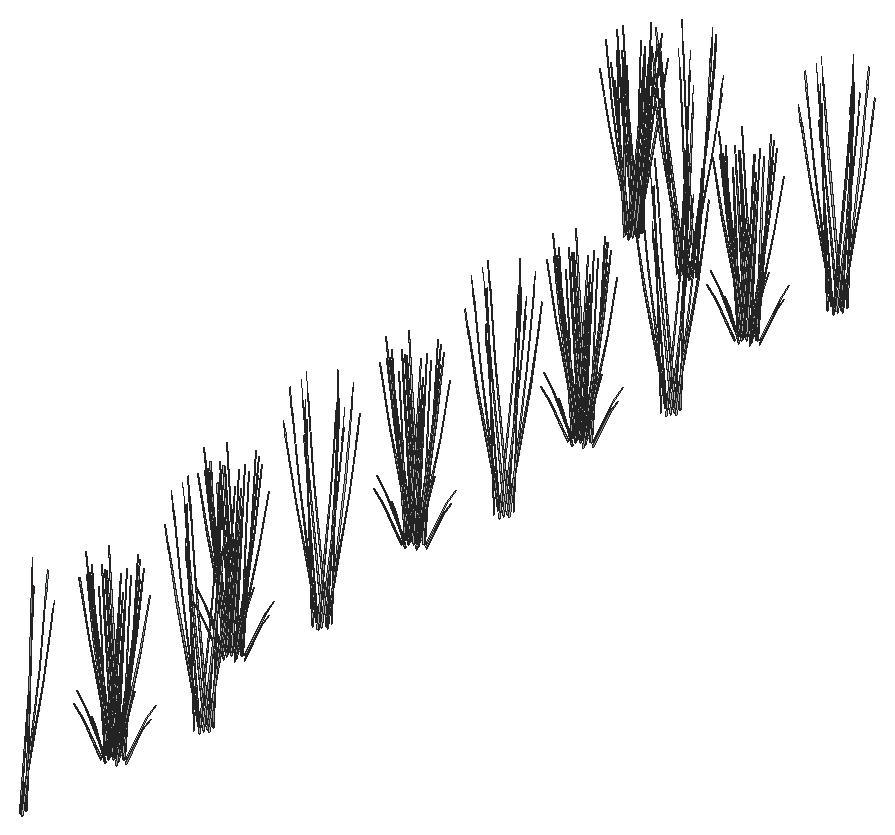
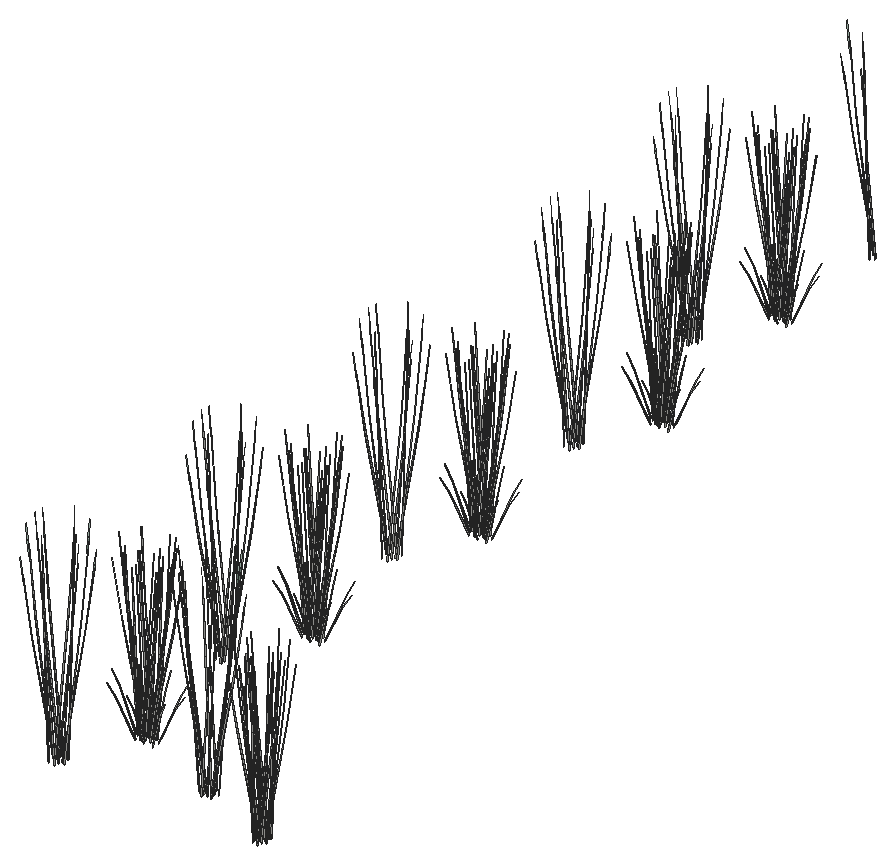
# SketchUp Ruby script. Lengths in inches.
U = 1.inch
M = Sketchup.active_model
def pt(a) = Geom::Point3d.new(a.map { |v| v * U })
def face(e, loops, mat)
  f = e.add_face(loops[0].map { |a| pt(a) })
  loops[1..].each { |l| e.add_face(l.map { |a| pt(a) }).erase! }
  f.material = f.back_material = mat if mat
  f
end
# faces: each face lists its corners as indices into pts; further lists are holes
def faces(e, pts, list, mat = nil) = list.each { |f| face(e, (f[0].is_a?(Array) ? f : [f]).map { |l| l.map { |i| pts[i] } }, mat) }
# xy, xz, yz: faces in a plane at the given z, y or x. An outline is a flat list of corners, or four numbers for a rectangle; further outlines are holes
def ring(l) = l.size == 4 ? [[l[0], l[1]], [l[2], l[1]], [l[2], l[3]], [l[0], l[3]]] : l.each_slice(2).to_a
def flat(e, list, mat, &to3) = list.each { |f| face(e, (f[0].is_a?(Array) ? f : [f]).map { |l| ring(l).map { |u, v| to3.(u, v) } }, mat) }
def xy(e, z, list, mat = nil) = flat(e, list, mat) { |x, y| [x, y, z] }
def xz(e, y, list, mat = nil) = flat(e, list, mat) { |x, z| [x, y, z] }
def yz(e, x, list, mat = nil) = flat(e, list, mat) { |y, z| [x, y, z] }
def lines(e, pts, list) = list.each { |a, b| e.add_line(pt(pts[a]), pt(pts[b])) }
# prism: a flat outline (further loops are holes) pulled along v
def prism(e, loops, v, mat = nil)
  f = face(e, loops, mat); d = Geom::Vector3d.new(v.map { |x| x * U })
  f.pushpull(f.normal.samedirection?(d) ? d.length : -d.length)
end
def box(e, o, s, mat = nil) = prism(e, [[o, [o[0] + s[0], o[1], o[2]], [o[0] + s[0], o[1] + s[1], o[2]], [o[0], o[1] + s[1], o[2]]]], [0, 0, s[2]], mat)
def at(x, y, z, deg = 0) = Geom::Transformation.translation(pt([x, y, z])) * Geom::Transformation.rotation(ORIGIN, Z_AXIS, deg.degrees)
def axes(o, x, y, z) = Geom::Transformation.new([*x, 0, *y, 0, *z, 0, *pt(o).to_a, 1])
def part(name) = M.definitions.add(name)
# library, detail: a bought-in or finely detailed component or shape, given as its bounding box
def library(name, o, s) = part(name).tap { |d| box(d.entities, o, s) }
def detail(e, o, s) = box(e.add_group.entities, o, s)
def put(e, d, t, mat = nil) = e.add_instance(d, t).tap { |i| i.material = mat if mat }
def group(e, t, mat = nil) = e.add_group.tap { |g| g.transformation = t; g.material = mat if mat }.entities
root = M.entities
M.materials.add("LightPink_Translucent").color = [175, 214, 192]
M.materials["LightPink_Translucent"].alpha = 0.75
c1 = part("blade")
p = [[2.15,0.21,22],[0,0.17,0],[0.09,0.45,0],[2.18,0.31,22],[2.29,0.31,22],[0.38,0.45,0],
  [2.48,0.24,33],[2.49,0.24,33],[2.48,0.22,33]]
faces(c1.entities,p,[[0,1,2,3],[4,5,2,3],[6,3,4,7],[8,0,3,6]])
c2 = part("seeds")
p = [[0.3,-0.1,1.38],[-0.01,-0.03,1.59],[-0.01,-0.03,0.03],[0.14,-0.07,-0.07],[0.29,-0.03,3],[0.15,0.01,3.11]]
faces(c2.entities,p,[[0,1,2,3],[1,0,4,5]],"LightPink_Translucent")
c3 = part("blade with seeds")
put(c3.entities,c1,at(0,0,0))
put(c3.entities,c2,axes([2.4,0.25,30.99],[1.5799,-0.05474,1.17369],[-0.12525,1.92788,0.29478],[-0.07173,-0.02425,1.56792]))
c4 = part("blade with seeds\#1")
put(c4.entities,c1,at(0,0,0))
put(root,c3,axes([494.75,325.05,139.01],[0.22267,0.44731,-0.45182],[-0.39927,0.26736,0],[0.05071,0.10188,1.43328]))
put(root,c3,axes([493.84,325.58,139.04],[0.33473,0.32192,-0.56741],[-0.30352,0.39991,-0.14892],[0.0835,0.129,1.25246]))
put(root,c3,axes([494.3,327.12,139.01],[-0.22267,0.44731,-0.45182],[-0.39927,-0.26736,0],[-0.05071,0.10188,1.43328]))
put(root,c3,axes([493.45,326.47,139.04],[-0.07301,0.49717,-0.56741],[-0.45037,-0.10491,-0.14892],[-0.05457,0.14837,1.25246]))
put(root,c4,axes([493.46,351.51,138.04],[-0.08339,0.01373,1.44662],[-0.46112,-0.15453,-0.221],[0.00774,-0.1289,0.24641]))
put(root,c4,axes([491.97,351.98,138.04],[-0.04815,0.0502,1.44662],[-0.48665,0.10822,-0.221],[-0.11756,-0.09845,0.24641]))
put(root,c4,axes([495.5,352.17,138.04],[-0.07441,-0.03002,1.44662],[-0.19113,-0.33536,-0.221],[0.12893,-0.09101,0.24641]))
put(root,c4,axes([492.77,353.36,138.53],[-0.20416,-0.39074,-0.57289],[0.5881,-0.14072,-0.15036],[-0.02257,-0.13232,1.26456]))
put(root,c4,axes([493.12,352.18,138.47],[0.46527,-0.19052,-0.40731],[0.2781,0.34163,0],[0.10597,-0.04339,1.29208]))
put(root,c4,axes([491.57,353.31,138.47],[0,-0.38104,-0.40731],[0.5562,0,0],[0,-0.08679,1.29208]))
put(root,c4,axes([493.67,352.96,138.5],[0.33485,-0.2864,-0.51151],[0.41596,0.2597,-0.13425],[0.13418,-0.07144,1.12907]))
put(root,c4,axes([493.08,353.47,138.625],[0.2412,-0.34335,-0.36702],[0.50118,0.16524,0.17663],[0,-0.07915,1.17838]))
put(root,c4,axes([491.81,353.32,138.48],[0.34702,-0.23774,-0.25413],[0.34702,0.23774,0.25413],[0,-0.07658,1.14007]))
put(root,c4,axes([493.22,352.33,138.48],[0.4638,0.09428,-0.25413],[-0.11678,0.33202,0.25413],[0.0935,-0.03829,1.14007]))
put(root,c4,axes([493.12,353.97,138.625],[-0.29864,-0.31983,-0.36702],[0.45236,-0.22522,0.17663],[-0.09664,-0.03957,1.17838]))
put(root,c4,axes([492.85,354.09,138.5],[-0.51713,-0.06247,-0.51151],[0.10913,-0.38535,-0.13425],[-0.15433,-0.04669,1.12907]))
put(root,c4,axes([496.56,353.61,138.04],[-0.02598,-0.05785,1.44662],[0.1802,-0.33839,-0.221],[0.18177,-0.00487,0.24641]))
put(root,c4,axes([491.19,353.55,138.04],[0.01261,0.06005,1.44662],[-0.25416,0.31361,-0.221],[-0.18053,-0.01581,0.24641]))
put(root,c4,axes([492.3,354.68,138.48],[-0.11678,-0.33202,-0.25413],[0.4638,-0.09428,0.25413],[-0.0935,-0.03829,1.14007]))
put(root,c4,axes([495.27,352.57,138.47],[0.46527,0.19052,-0.40731],[-0.2781,0.34163,0],[0.10597,0.04339,1.29208]))
put(root,c4,axes([492.17,354.82,138.47],[-0.46527,-0.19052,-0.40731],[0.2781,-0.34163,0],[-0.10597,-0.04339,1.29208]))
put(root,c4,axes([495.14,352.71,138.48],[0.11678,0.33202,-0.25413],[-0.4638,0.09428,0.25413],[0.0935,0.03829,1.14007]))
put(root,c4,axes([494.59,353.3,138.5],[0.51713,0.06247,-0.51151],[-0.10913,0.38535,-0.13425],[0.15433,0.04669,1.12907]))
put(root,c4,axes([494.32,353.42,138.625],[0.29864,0.31983,-0.36702],[-0.45236,0.22522,0.17663],[0.09664,0.03957,1.17838]))
put(root,c4,axes([493.76,354.2,138.625],[-0.53984,0.02352,-0.36702],[-0.04882,-0.39046,0.17663],[-0.09664,0.03957,1.17838]))
put(root,c4,axes([494.22,355.06,138.48],[-0.4638,-0.09428,-0.25413],[0.11678,-0.33202,0.25413],[-0.0935,0.03829,1.14007]))
put(root,c4,axes([495.63,354.07,138.48],[-0.34702,0.23774,-0.25413],[-0.34702,-0.23774,0.25413],[0,0.07658,1.14007]))
put(root,c4,axes([494.36,353.92,138.625],[-0.2412,0.34335,-0.36702],[-0.50118,-0.16524,0.17663],[0,0.07915,1.17838]))
put(root,c4,axes([493.77,354.43,138.5],[-0.33485,0.2864,-0.51151],[-0.41596,-0.2597,-0.13425],[-0.13418,0.07144,1.12907]))
put(root,c4,axes([495.87,354.08,138.47],[0,0.38104,-0.40731],[-0.5562,0,0],[0,0.08679,1.29208]))
put(root,c4,axes([494.32,355.21,138.47],[-0.46527,0.19052,-0.40731],[-0.2781,-0.34163,0],[-0.10597,0.04339,1.29208]))
put(root,c4,axes([494.64,354.03,138.53],[0.18229,0.34888,-0.56778],[-0.52509,0.12565,-0.14902],[0.02015,0.11814,1.25327]))
put(root,c4,axes([495.24,355.28,138.04],[0.03622,-0.05501,1.44662],[0.45599,-0.16202,-0.221],[0.13824,0.08385,0.24641]))
put(root,c4,axes([491.05,355.23,138.04],[0.06668,0.03807,1.44662],[0.11307,0.35272,-0.221],[-0.14779,0.07522,0.24641]))
put(root,c4,axes([493.11,355.27,138.04],[0.08046,-0.02073,1.44662],[0.48396,0.11412,-0.221],[0.01415,0.12863,0.24641]))
put(root,c3,axes([499.96,370.71,139.14],[0.07301,-0.49717,-0.56741],[0.45037,0.10491,-0.14892],[0.05457,-0.14837,1.25246]))
put(root,c3,axes([499.11,370.06,139.1],[0.22267,-0.44731,-0.45182],[0.39927,0.26736,0],[0.05071,-0.10188,1.43328]))
put(root,c3,axes([499.57,371.59,139.14],[-0.33473,-0.32192,-0.56741],[0.30352,-0.39991,-0.14892],[-0.0835,-0.129,1.25246]))
put(root,c3,axes([498.66,372.12,139.1],[-0.22267,-0.44731,-0.45182],[0.39927,-0.26736,0],[-0.05071,-0.10188,1.43328]))
put(root,c3,axes([500.875,369.47,139.1],[0.44533,0,-0.45182],[0,0.53472,0],[0.10143,0,1.43328]))
put(root,c3,axes([500.81,370.63,139.17],[0.45667,-0.19628,-0.6355],[0.16447,0.5654,-0.16679],[0.15464,-0.02169,1.40276]))
put(root,c3,axes([500.03,372.43,139.17],[-0.40774,0.17525,-0.62983],[-0.14685,-0.50482,-0.1653],[-0.13807,0.01937,1.39023]))
put(root,c3,axes([499.97,373.61,139.1],[-0.44533,0,-0.45182],[0,-0.53472,0],[-0.10143,0,1.43328]))
put(root,c3,axes([502.19,370.96,139.1],[0.22267,0.44731,-0.45182],[-0.39927,0.26736,0],[0.05071,0.10188,1.43328]))
put(root,c3,axes([501.28,371.49,139.14],[0.33473,0.32192,-0.56741],[-0.30352,0.39991,-0.14892],[0.0835,0.129,1.25246]))
put(root,c3,axes([501.74,373.03,139.1],[-0.22267,0.44731,-0.45182],[-0.39927,-0.26736,0],[-0.05071,0.10188,1.43328]))
put(root,c3,axes([500.89,372.375,139.14],[-0.07301,0.49717,-0.56741],[-0.45037,-0.10491,-0.14892],[-0.05457,0.14837,1.25246]))
put(root,c4,axes([486.02,395.73,137.94],[-0.08339,0.01373,1.44662],[-0.46112,-0.15453,-0.221],[0.00774,-0.1289,0.24641]))
put(root,c4,axes([484.53,396.2,137.94],[-0.04815,0.0502,1.44662],[-0.48665,0.10822,-0.221],[-0.11756,-0.09845,0.24641]))
put(root,c4,axes([488.0625,396.38,137.94],[-0.07441,-0.03002,1.44662],[-0.19113,-0.33536,-0.221],[0.12893,-0.09101,0.24641]))
put(root,c4,axes([485.33,397.58,138.4375],[-0.20416,-0.39074,-0.57289],[0.5881,-0.14072,-0.15036],[-0.02257,-0.13232,1.26456]))
put(root,c4,axes([485.67,396.39,138.37],[0.46527,-0.19052,-0.40731],[0.2781,0.34163,0],[0.10597,-0.04339,1.29208]))
put(root,c4,axes([484.13,397.52,138.37],[0,-0.38104,-0.40731],[0.5562,0,0],[0,-0.08679,1.29208]))
put(root,c4,axes([486.22,397.18,138.41],[0.33485,-0.2864,-0.51151],[0.41596,0.2597,-0.13425],[0.13418,-0.07144,1.12907]))
put(root,c4,axes([485.64,397.68,138.53],[0.2412,-0.34335,-0.36702],[0.50118,0.16524,0.17663],[0,-0.07915,1.17838]))
put(root,c4,axes([484.37,397.53,138.38],[0.34702,-0.23774,-0.25413],[0.34702,0.23774,0.25413],[0,-0.07658,1.14007]))
put(root,c4,axes([485.78,396.55,138.38],[0.4638,0.09428,-0.25413],[-0.11678,0.33202,0.25413],[0.0935,-0.03829,1.14007]))
put(root,c4,axes([485.68,398.18,138.53],[-0.29864,-0.31983,-0.36702],[0.45236,-0.22522,0.17663],[-0.09664,-0.03957,1.17838]))
put(root,c4,axes([485.41,398.31,138.41],[-0.51713,-0.06247,-0.51151],[0.10913,-0.38535,-0.13425],[-0.15433,-0.04669,1.12907]))
put(root,c4,axes([489.11,397.82,137.94],[-0.02598,-0.05785,1.44662],[0.1802,-0.33839,-0.221],[0.18177,-0.00487,0.24641]))
put(root,c4,axes([483.75,397.76,137.94],[0.01261,0.06005,1.44662],[-0.25416,0.31361,-0.221],[-0.18053,-0.01581,0.24641]))
put(root,c4,axes([484.86,398.89,138.38],[-0.11678,-0.33202,-0.25413],[0.4638,-0.09428,0.25413],[-0.0935,-0.03829,1.14007]))
put(root,c4,axes([487.82,396.78,138.37],[0.46527,0.19052,-0.40731],[-0.2781,0.34163,0],[0.10597,0.04339,1.29208]))
put(root,c4,axes([484.73,399.04,138.37],[-0.46527,-0.19052,-0.40731],[0.2781,-0.34163,0],[-0.10597,-0.04339,1.29208]))
put(root,c4,axes([487.69,396.92,138.38],[0.11678,0.33202,-0.25413],[-0.4638,0.09428,0.25413],[0.0935,0.03829,1.14007]))
put(root,c4,axes([487.14,397.51,138.41],[0.51713,0.06247,-0.51151],[-0.10913,0.38535,-0.13425],[0.15433,0.04669,1.12907]))
put(root,c4,axes([486.875,397.63,138.53],[0.29864,0.31983,-0.36702],[-0.45236,0.22522,0.17663],[0.09664,0.03957,1.17838]))
put(root,c4,axes([486.32,398.41,138.53],[-0.53984,0.02352,-0.36702],[-0.04882,-0.39046,0.17663],[-0.09664,0.03957,1.17838]))
put(root,c4,axes([486.77,399.27,138.38],[-0.4638,-0.09428,-0.25413],[0.11678,-0.33202,0.25413],[-0.0935,0.03829,1.14007]))
put(root,c4,axes([488.1875,398.28,138.38],[-0.34702,0.23774,-0.25413],[-0.34702,-0.23774,0.25413],[0,0.07658,1.14007]))
put(root,c4,axes([486.91,398.14,138.53],[-0.2412,0.34335,-0.36702],[-0.50118,-0.16524,0.17663],[0,0.07915,1.17838]))
put(root,c4,axes([486.33,398.64,138.41],[-0.33485,0.2864,-0.51151],[-0.41596,-0.2597,-0.13425],[-0.13418,0.07144,1.12907]))
put(root,c4,axes([488.43,398.29,138.37],[0,0.38104,-0.40731],[-0.5562,0,0],[0,0.08679,1.29208]))
put(root,c4,axes([486.88,399.42,138.37],[-0.46527,0.19052,-0.40731],[-0.2781,-0.34163,0],[-0.10597,0.04339,1.29208]))
put(root,c4,axes([487.2,398.24,138.4375],[0.18229,0.34888,-0.56778],[-0.52509,0.12565,-0.14902],[0.02015,0.11814,1.25327]))
put(root,c4,axes([487.8,399.49,137.94],[0.03622,-0.05501,1.44662],[0.45599,-0.16202,-0.221],[0.13824,0.08385,0.24641]))
put(root,c4,axes([483.61,399.44,137.94],[0.06668,0.03807,1.44662],[0.11307,0.35272,-0.221],[-0.14779,0.07522,0.24641]))
put(root,c4,axes([485.67,399.48,137.94],[0.08046,-0.02073,1.44662],[0.48396,0.11412,-0.221],[0.01415,0.12863,0.24641]))
put(root,c3,axes([492.52,414.92,139.04],[0.07301,-0.49717,-0.56741],[0.45037,0.10491,-0.14892],[0.05457,-0.14837,1.25246]))
put(root,c3,axes([491.66,414.27,139.01],[0.22267,-0.44731,-0.45182],[0.39927,0.26736,0],[0.05071,-0.10188,1.43328]))
put(root,c3,axes([492.125,415.81,139.04],[-0.33473,-0.32192,-0.56741],[0.30352,-0.39991,-0.14892],[-0.0835,-0.129,1.25246]))
put(root,c3,axes([491.21,416.34,139.01],[-0.22267,-0.44731,-0.45182],[0.39927,-0.26736,0],[-0.05071,-0.10188,1.43328]))
put(root,c3,axes([493.43,413.6875,139.01],[0.44533,0,-0.45182],[0,0.53472,0],[0.10143,0,1.43328]))
put(root,c3,axes([493.37,414.84,139.08],[0.45667,-0.19628,-0.6355],[0.16447,0.5654,-0.16679],[0.15464,-0.02169,1.40276]))
put(root,c3,axes([492.59,416.64,139.08],[-0.40774,0.17525,-0.62983],[-0.14685,-0.50482,-0.1653],[-0.13807,0.01937,1.39023]))
put(root,c3,axes([492.53,417.82,139.01],[-0.44533,0,-0.45182],[0,-0.53472,0],[-0.10143,0,1.43328]))
put(root,c3,axes([494.75,415.17,139.01],[0.22267,0.44731,-0.45182],[-0.39927,0.26736,0],[0.05071,0.10188,1.43328]))
put(root,c3,axes([493.84,415.7,139.04],[0.33473,0.32192,-0.56741],[-0.30352,0.39991,-0.14892],[0.0835,0.129,1.25246]))
put(root,c3,axes([494.3,417.24,139.01],[-0.22267,0.44731,-0.45182],[-0.39927,-0.26736,0],[-0.05071,0.10188,1.43328]))
put(root,c3,axes([493.45,416.59,139.04],[-0.07301,0.49717,-0.56741],[-0.45037,-0.10491,-0.14892],[-0.05457,0.14837,1.25246]))
put(root,c4,axes([486.02,449.3,137.94],[-0.08339,0.01373,1.44662],[-0.46112,-0.15453,-0.221],[0.00774,-0.1289,0.24641]))
put(root,c4,axes([484.53,449.77,137.94],[-0.04815,0.0502,1.44662],[-0.48665,0.10822,-0.221],[-0.11756,-0.09845,0.24641]))
put(root,c4,axes([488.0625,449.96,137.94],[-0.07441,-0.03002,1.44662],[-0.19113,-0.33536,-0.221],[0.12893,-0.09101,0.24641]))
put(root,c4,axes([485.33,451.15,138.4375],[-0.20416,-0.39074,-0.57289],[0.5881,-0.14072,-0.15036],[-0.02257,-0.13232,1.26456]))
put(root,c4,axes([485.67,449.97,138.37],[0.46527,-0.19052,-0.40731],[0.2781,0.34163,0],[0.10597,-0.04339,1.29208]))
put(root,c4,axes([484.13,451.1,138.37],[0,-0.38104,-0.40731],[0.5562,0,0],[0,-0.08679,1.29208]))
put(root,c4,axes([486.22,450.75,138.41],[0.33485,-0.2864,-0.51151],[0.41596,0.2597,-0.13425],[0.13418,-0.07144,1.12907]))
put(root,c4,axes([485.64,451.25,138.53],[0.2412,-0.34335,-0.36702],[0.50118,0.16524,0.17663],[0,-0.07915,1.17838]))
put(root,c4,axes([484.37,451.1,138.38],[0.34702,-0.23774,-0.25413],[0.34702,0.23774,0.25413],[0,-0.07658,1.14007]))
put(root,c4,axes([485.78,450.12,138.38],[0.4638,0.09428,-0.25413],[-0.11678,0.33202,0.25413],[0.0935,-0.03829,1.14007]))
put(root,c4,axes([485.68,451.76,138.53],[-0.29864,-0.31983,-0.36702],[0.45236,-0.22522,0.17663],[-0.09664,-0.03957,1.17838]))
put(root,c4,axes([485.41,451.88,138.41],[-0.51713,-0.06247,-0.51151],[0.10913,-0.38535,-0.13425],[-0.15433,-0.04669,1.12907]))
put(root,c4,axes([489.11,451.39,137.94],[-0.02598,-0.05785,1.44662],[0.1802,-0.33839,-0.221],[0.18177,-0.00487,0.24641]))
put(root,c4,axes([483.75,451.34,137.94],[0.01261,0.06005,1.44662],[-0.25416,0.31361,-0.221],[-0.18053,-0.01581,0.24641]))
put(root,c4,axes([484.86,452.47,138.38],[-0.11678,-0.33202,-0.25413],[0.4638,-0.09428,0.25413],[-0.0935,-0.03829,1.14007]))
put(root,c4,axes([487.82,450.35,138.37],[0.46527,0.19052,-0.40731],[-0.2781,0.34163,0],[0.10597,0.04339,1.29208]))
put(root,c4,axes([484.73,452.61,138.37],[-0.46527,-0.19052,-0.40731],[0.2781,-0.34163,0],[-0.10597,-0.04339,1.29208]))
put(root,c4,axes([487.69,450.5,138.38],[0.11678,0.33202,-0.25413],[-0.4638,0.09428,0.25413],[0.0935,0.03829,1.14007]))
put(root,c4,axes([487.14,451.08,138.41],[0.51713,0.06247,-0.51151],[-0.10913,0.38535,-0.13425],[0.15433,0.04669,1.12907]))
put(root,c4,axes([486.875,451.21,138.53],[0.29864,0.31983,-0.36702],[-0.45236,0.22522,0.17663],[0.09664,0.03957,1.17838]))
put(root,c4,axes([486.32,451.99,138.53],[-0.53984,0.02352,-0.36702],[-0.04882,-0.39046,0.17663],[-0.09664,0.03957,1.17838]))
put(root,c4,axes([486.77,452.84,138.38],[-0.4638,-0.09428,-0.25413],[0.11678,-0.33202,0.25413],[-0.0935,0.03829,1.14007]))
put(root,c4,axes([488.1875,451.86,138.38],[-0.34702,0.23774,-0.25413],[-0.34702,-0.23774,0.25413],[0,0.07658,1.14007]))
put(root,c4,axes([486.91,451.71,138.53],[-0.2412,0.34335,-0.36702],[-0.50118,-0.16524,0.17663],[0,0.07915,1.17838]))
put(root,c4,axes([486.33,452.21,138.41],[-0.33485,0.2864,-0.51151],[-0.41596,-0.2597,-0.13425],[-0.13418,0.07144,1.12907]))
put(root,c4,axes([488.43,451.87,138.37],[0,0.38104,-0.40731],[-0.5562,0,0],[0,0.08679,1.29208]))
put(root,c4,axes([486.88,452.99,138.37],[-0.46527,0.19052,-0.40731],[-0.2781,-0.34163,0],[-0.10597,0.04339,1.29208]))
put(root,c4,axes([487.2,451.81,138.4375],[0.18229,0.34888,-0.56778],[-0.52509,0.12565,-0.14902],[0.02015,0.11814,1.25327]))
put(root,c4,axes([487.8,453.0625,137.94],[0.03622,-0.05501,1.44662],[0.45599,-0.16202,-0.221],[0.13824,0.08385,0.24641]))
put(root,c4,axes([483.61,453.02,137.94],[0.06668,0.03807,1.44662],[0.11307,0.35272,-0.221],[-0.14779,0.07522,0.24641]))
put(root,c4,axes([485.67,453.05,137.94],[0.08046,-0.02073,1.44662],[0.48396,0.11412,-0.221],[0.01415,0.12863,0.24641]))
put(root,c3,axes([492.52,468.49,139.04],[0.07301,-0.49717,-0.56741],[0.45037,0.10491,-0.14892],[0.05457,-0.14837,1.25246]))
put(root,c3,axes([491.66,467.84,139.01],[0.22267,-0.44731,-0.45182],[0.39927,0.26736,0],[0.05071,-0.10188,1.43328]))
put(root,c3,axes([492.125,469.38,139.04],[-0.33473,-0.32192,-0.56741],[0.30352,-0.39991,-0.14892],[-0.0835,-0.129,1.25246]))
put(root,c3,axes([491.21,469.91,139.01],[-0.22267,-0.44731,-0.45182],[0.39927,-0.26736,0],[-0.05071,-0.10188,1.43328]))
put(root,c3,axes([493.43,467.26,139.01],[0.44533,0,-0.45182],[0,0.53472,0],[0.10143,0,1.43328]))
put(root,c3,axes([493.37,468.42,139.08],[0.45667,-0.19628,-0.6355],[0.16447,0.5654,-0.16679],[0.15464,-0.02169,1.40276]))
put(root,c3,axes([492.59,470.21,139.08],[-0.40774,0.17525,-0.62983],[-0.14685,-0.50482,-0.1653],[-0.13807,0.01937,1.39023]))
put(root,c3,axes([492.53,471.4,139.01],[-0.44533,0,-0.45182],[0,-0.53472,0],[-0.10143,0,1.43328]))
put(root,c3,axes([494.75,468.75,139.01],[0.22267,0.44731,-0.45182],[-0.39927,0.26736,0],[0.05071,0.10188,1.43328]))
put(root,c3,axes([493.84,469.28,139.04],[0.33473,0.32192,-0.56741],[-0.30352,0.39991,-0.14892],[0.0835,0.129,1.25246]))
put(root,c3,axes([494.3,470.8125,139.01],[-0.22267,0.44731,-0.45182],[-0.39927,-0.26736,0],[-0.05071,0.10188,1.43328]))
put(root,c3,axes([493.45,470.16,139.04],[-0.07301,0.49717,-0.56741],[-0.45037,-0.10491,-0.14892],[-0.05457,0.14837,1.25246]))
put(root,c4,axes([486.02,498.51,137.94],[-0.08339,0.01373,1.44662],[-0.46112,-0.15453,-0.221],[0.00774,-0.1289,0.24641]))
put(root,c4,axes([484.53,498.98,137.94],[-0.04815,0.0502,1.44662],[-0.48665,0.10822,-0.221],[-0.11756,-0.09845,0.24641]))
put(root,c4,axes([488.0625,499.17,137.94],[-0.07441,-0.03002,1.44662],[-0.19113,-0.33536,-0.221],[0.12893,-0.09101,0.24641]))
put(root,c4,axes([485.33,500.36,138.4375],[-0.20416,-0.39074,-0.57289],[0.5881,-0.14072,-0.15036],[-0.02257,-0.13232,1.26456]))
put(root,c4,axes([485.67,499.18,138.37],[0.46527,-0.19052,-0.40731],[0.2781,0.34163,0],[0.10597,-0.04339,1.29208]))
put(root,c4,axes([484.13,500.31,138.37],[0,-0.38104,-0.40731],[0.5562,0,0],[0,-0.08679,1.29208]))
put(root,c4,axes([486.22,499.96,138.41],[0.33485,-0.2864,-0.51151],[0.41596,0.2597,-0.13425],[0.13418,-0.07144,1.12907]))
put(root,c4,axes([485.64,500.46,138.53],[0.2412,-0.34335,-0.36702],[0.50118,0.16524,0.17663],[0,-0.07915,1.17838]))
put(root,c4,axes([484.37,500.3125,138.38],[0.34702,-0.23774,-0.25413],[0.34702,0.23774,0.25413],[0,-0.07658,1.14007]))
put(root,c4,axes([485.78,499.33,138.38],[0.4638,0.09428,-0.25413],[-0.11678,0.33202,0.25413],[0.0935,-0.03829,1.14007]))
put(root,c4,axes([485.68,500.97,138.53],[-0.29864,-0.31983,-0.36702],[0.45236,-0.22522,0.17663],[-0.09664,-0.03957,1.17838]))
put(root,c4,axes([485.41,501.09,138.41],[-0.51713,-0.06247,-0.51151],[0.10913,-0.38535,-0.13425],[-0.15433,-0.04669,1.12907]))
put(root,c4,axes([489.11,500.6,137.94],[-0.02598,-0.05785,1.44662],[0.1802,-0.33839,-0.221],[0.18177,-0.00487,0.24641]))
put(root,c4,axes([483.75,500.54,137.94],[0.01261,0.06005,1.44662],[-0.25416,0.31361,-0.221],[-0.18053,-0.01581,0.24641]))
put(root,c4,axes([484.86,501.68,138.38],[-0.11678,-0.33202,-0.25413],[0.4638,-0.09428,0.25413],[-0.0935,-0.03829,1.14007]))
put(root,c4,axes([487.82,499.5625,138.37],[0.46527,0.19052,-0.40731],[-0.2781,0.34163,0],[0.10597,0.04339,1.29208]))
put(root,c4,axes([484.73,501.82,138.37],[-0.46527,-0.19052,-0.40731],[0.2781,-0.34163,0],[-0.10597,-0.04339,1.29208]))
put(root,c4,axes([487.69,499.71,138.38],[0.11678,0.33202,-0.25413],[-0.4638,0.09428,0.25413],[0.0935,0.03829,1.14007]))
put(root,c4,axes([487.14,500.29,138.41],[0.51713,0.06247,-0.51151],[-0.10913,0.38535,-0.13425],[0.15433,0.04669,1.12907]))
put(root,c4,axes([486.875,500.41,138.53],[0.29864,0.31983,-0.36702],[-0.45236,0.22522,0.17663],[0.09664,0.03957,1.17838]))
put(root,c4,axes([486.32,501.2,138.53],[-0.53984,0.02352,-0.36702],[-0.04882,-0.39046,0.17663],[-0.09664,0.03957,1.17838]))
put(root,c4,axes([486.77,502.05,138.38],[-0.4638,-0.09428,-0.25413],[0.11678,-0.33202,0.25413],[-0.0935,0.03829,1.14007]))
put(root,c4,axes([488.1875,501.07,138.38],[-0.34702,0.23774,-0.25413],[-0.34702,-0.23774,0.25413],[0,0.07658,1.14007]))
put(root,c4,axes([486.91,500.92,138.53],[-0.2412,0.34335,-0.36702],[-0.50118,-0.16524,0.17663],[0,0.07915,1.17838]))
put(root,c4,axes([486.33,501.42,138.41],[-0.33485,0.2864,-0.51151],[-0.41596,-0.2597,-0.13425],[-0.13418,0.07144,1.12907]))
put(root,c4,axes([488.43,501.08,138.37],[0,0.38104,-0.40731],[-0.5562,0,0],[0,0.08679,1.29208]))
put(root,c4,axes([486.88,502.2,138.37],[-0.46527,0.19052,-0.40731],[-0.2781,-0.34163,0],[-0.10597,0.04339,1.29208]))
put(root,c4,axes([487.2,501.02,138.4375],[0.18229,0.34888,-0.56778],[-0.52509,0.12565,-0.14902],[0.02015,0.11814,1.25327]))
put(root,c4,axes([487.8,502.27,137.94],[0.03622,-0.05501,1.44662],[0.45599,-0.16202,-0.221],[0.13824,0.08385,0.24641]))
put(root,c4,axes([483.61,502.23,137.94],[0.06668,0.03807,1.44662],[0.11307,0.35272,-0.221],[-0.14779,0.07522,0.24641]))
put(root,c4,axes([485.67,502.26,137.94],[0.08046,-0.02073,1.44662],[0.48396,0.11412,-0.221],[0.01415,0.12863,0.24641]))
put(root,c3,axes([492.52,517.7,139.04],[0.07301,-0.49717,-0.56741],[0.45037,0.10491,-0.14892],[0.05457,-0.14837,1.25246]))
put(root,c3,axes([491.66,517.05,139.01],[0.22267,-0.44731,-0.45182],[0.39927,0.26736,0],[0.05071,-0.10188,1.43328]))
put(root,c3,axes([492.125,518.59,139.04],[-0.33473,-0.32192,-0.56741],[0.30352,-0.39991,-0.14892],[-0.0835,-0.129,1.25246]))
put(root,c3,axes([491.21,519.12,139.01],[-0.22267,-0.44731,-0.45182],[0.39927,-0.26736,0],[-0.05071,-0.10188,1.43328]))
put(root,c3,axes([493.43,516.47,139.01],[0.44533,0,-0.45182],[0,0.53472,0],[0.10143,0,1.43328]))
put(root,c3,axes([493.37,517.63,139.08],[0.45667,-0.19628,-0.6355],[0.16447,0.5654,-0.16679],[0.15464,-0.02169,1.40276]))
put(root,c3,axes([492.59,519.42,139.08],[-0.40774,0.17525,-0.62983],[-0.14685,-0.50482,-0.1653],[-0.13807,0.01937,1.39023]))
put(root,c3,axes([492.53,520.6,139.01],[-0.44533,0,-0.45182],[0,-0.53472,0],[-0.10143,0,1.43328]))
put(root,c3,axes([494.75,517.96,139.01],[0.22267,0.44731,-0.45182],[-0.39927,0.26736,0],[0.05071,0.10188,1.43328]))
put(root,c3,axes([493.84,518.49,139.04],[0.33473,0.32192,-0.56741],[-0.30352,0.39991,-0.14892],[0.0835,0.129,1.25246]))
put(root,c3,axes([494.3,520.02,139.01],[-0.22267,0.44731,-0.45182],[-0.39927,-0.26736,0],[-0.05071,0.10188,1.43328]))
put(root,c3,axes([493.45,519.37,139.04],[-0.07301,0.49717,-0.56741],[-0.45037,-0.10491,-0.14892],[-0.05457,0.14837,1.25246]))
put(root,c4,axes([486.02,547.56,137.94],[-0.08339,0.01373,1.44662],[-0.46112,-0.15453,-0.221],[0.00774,-0.1289,0.24641]))
put(root,c4,axes([484.53,548.03,137.94],[-0.04815,0.0502,1.44662],[-0.48665,0.10822,-0.221],[-0.11756,-0.09845,0.24641]))
put(root,c4,axes([488.0625,548.22,137.94],[-0.07441,-0.03002,1.44662],[-0.19113,-0.33536,-0.221],[0.12893,-0.09101,0.24641]))
put(root,c4,axes([485.33,549.41,138.4375],[-0.20416,-0.39074,-0.57289],[0.5881,-0.14072,-0.15036],[-0.02257,-0.13232,1.26456]))
put(root,c4,axes([485.67,548.23,138.37],[0.46527,-0.19052,-0.40731],[0.2781,0.34163,0],[0.10597,-0.04339,1.29208]))
put(root,c4,axes([484.13,549.35,138.37],[0,-0.38104,-0.40731],[0.5562,0,0],[0,-0.08679,1.29208]))
put(root,c4,axes([486.22,549.01,138.41],[0.33485,-0.2864,-0.51151],[0.41596,0.2597,-0.13425],[0.13418,-0.07144,1.12907]))
put(root,c4,axes([485.64,549.51,138.53],[0.2412,-0.34335,-0.36702],[0.50118,0.16524,0.17663],[0,-0.07915,1.17838]))
put(root,c4,axes([484.37,549.36,138.38],[0.34702,-0.23774,-0.25413],[0.34702,0.23774,0.25413],[0,-0.07658,1.14007]))
put(root,c4,axes([485.78,548.38,138.38],[0.4638,0.09428,-0.25413],[-0.11678,0.33202,0.25413],[0.0935,-0.03829,1.14007]))
put(root,c4,axes([485.68,550.02,138.53],[-0.29864,-0.31983,-0.36702],[0.45236,-0.22522,0.17663],[-0.09664,-0.03957,1.17838]))
put(root,c4,axes([485.41,550.14,138.41],[-0.51713,-0.06247,-0.51151],[0.10913,-0.38535,-0.13425],[-0.15433,-0.04669,1.12907]))
put(root,c4,axes([489.11,549.65,137.94],[-0.02598,-0.05785,1.44662],[0.1802,-0.33839,-0.221],[0.18177,-0.00487,0.24641]))
put(root,c4,axes([483.75,549.59,137.94],[0.01261,0.06005,1.44662],[-0.25416,0.31361,-0.221],[-0.18053,-0.01581,0.24641]))
put(root,c4,axes([484.86,550.73,138.38],[-0.11678,-0.33202,-0.25413],[0.4638,-0.09428,0.25413],[-0.0935,-0.03829,1.14007]))
put(root,c4,axes([487.82,548.61,138.37],[0.46527,0.19052,-0.40731],[-0.2781,0.34163,0],[0.10597,0.04339,1.29208]))
put(root,c4,axes([484.73,550.87,138.37],[-0.46527,-0.19052,-0.40731],[0.2781,-0.34163,0],[-0.10597,-0.04339,1.29208]))
put(root,c4,axes([487.69,548.75,138.38],[0.11678,0.33202,-0.25413],[-0.4638,0.09428,0.25413],[0.0935,0.03829,1.14007]))
put(root,c4,axes([487.14,549.34,138.41],[0.51713,0.06247,-0.51151],[-0.10913,0.38535,-0.13425],[0.15433,0.04669,1.12907]))
put(root,c4,axes([486.875,549.46,138.53],[0.29864,0.31983,-0.36702],[-0.45236,0.22522,0.17663],[0.09664,0.03957,1.17838]))
put(root,c4,axes([486.32,550.25,138.53],[-0.53984,0.02352,-0.36702],[-0.04882,-0.39046,0.17663],[-0.09664,0.03957,1.17838]))
put(root,c4,axes([486.77,551.1,138.38],[-0.4638,-0.09428,-0.25413],[0.11678,-0.33202,0.25413],[-0.0935,0.03829,1.14007]))
put(root,c4,axes([488.1875,550.12,138.38],[-0.34702,0.23774,-0.25413],[-0.34702,-0.23774,0.25413],[0,0.07658,1.14007]))
put(root,c4,axes([486.91,549.97,138.53],[-0.2412,0.34335,-0.36702],[-0.50118,-0.16524,0.17663],[0,0.07915,1.17838]))
put(root,c4,axes([486.33,550.47,138.41],[-0.33485,0.2864,-0.51151],[-0.41596,-0.2597,-0.13425],[-0.13418,0.07144,1.12907]))
put(root,c4,axes([488.43,550.125,138.37],[0,0.38104,-0.40731],[-0.5562,0,0],[0,0.08679,1.29208]))
put(root,c4,axes([486.88,551.25,138.37],[-0.46527,0.19052,-0.40731],[-0.2781,-0.34163,0],[-0.10597,0.04339,1.29208]))
put(root,c4,axes([487.2,550.07,138.4375],[0.18229,0.34888,-0.56778],[-0.52509,0.12565,-0.14902],[0.02015,0.11814,1.25327]))
put(root,c4,axes([487.8,551.32,137.94],[0.03622,-0.05501,1.44662],[0.45599,-0.16202,-0.221],[0.13824,0.08385,0.24641]))
put(root,c4,axes([483.61,551.28,137.94],[0.06668,0.03807,1.44662],[0.11307,0.35272,-0.221],[-0.14779,0.07522,0.24641]))
put(root,c4,axes([485.67,551.31,137.94],[0.08046,-0.02073,1.44662],[0.48396,0.11412,-0.221],[0.01415,0.12863,0.24641]))
put(root,c3,axes([462.53,559.7,139.17],[-0.19628,-0.45667,-0.6355],[0.5654,-0.16447,-0.16679],[-0.02169,-0.15464,1.40276]))
put(root,c3,axes([461.38,559.64,139.1],[0,-0.44533,-0.45182],[0.53472,0,0],[0,-0.10143,1.43328]))
put(root,c3,axes([462.86,558.32,139.1],[0.44731,-0.22267,-0.45182],[0.26736,0.39927,0],[0.10188,-0.05071,1.43328]))
put(root,c3,axes([463.39,559.23,139.14],[0.32192,-0.33473,-0.56741],[0.39991,0.30352,-0.14892],[0.129,-0.0835,1.25246]))
put(root,c3,axes([462.61,560.56,139.14],[-0.49717,-0.07301,-0.56741],[0.10491,-0.45037,-0.14892],[-0.14837,-0.05457,1.25246]))
put(root,c3,axes([461.96,561.41,139.1],[-0.44731,-0.22267,-0.45182],[0.26736,-0.39927,0],[-0.10188,-0.05071,1.43328]))
put(root,c3,axes([464.93,558.77,139.1],[0.44731,0.22267,-0.45182],[-0.26736,0.39927,0],[0.10188,0.05071,1.43328]))
put(root,c3,axes([464.28,559.625,139.14],[0.49717,0.07301,-0.56741],[-0.10491,0.45037,-0.14892],[0.14837,0.05457,1.25246]))
put(root,c4,axes([445.2,565.93,138.5],[0.06247,-0.51713,-0.51151],[0.38535,0.10913,-0.13425],[0.04669,-0.15433,1.12907]))
put(root,c3,axes([463.5,560.94,139.14],[-0.32192,0.33473,-0.56741],[-0.39991,-0.30352,-0.14892],[-0.129,0.0835,1.25246]))
put(root,c4,axes([444.47,565.25,138.47],[0.19052,-0.46527,-0.40731],[0.34163,0.2781,0],[0.04339,-0.10597,1.29208]))
put(root,c3,axes([464.03,561.86,139.1],[-0.44731,0.22267,-0.45182],[-0.26736,-0.39927,0],[-0.10188,0.05071,1.43328]))
put(root,c3,axes([465.51,560.54,139.1],[0,0.44533,-0.45182],[-0.53472,0,0],[0,0.10143,1.43328]))
put(root,c3,axes([492.52,566.75,139.04],[0.07301,-0.49717,-0.56741],[0.45037,0.10491,-0.14892],[0.05457,-0.14837,1.25246]))
put(root,c3,axes([464.33,560.48,139.17],[0.17525,0.40774,-0.62983],[-0.50482,0.14685,-0.1653],[0.01937,0.13807,1.39023]))
put(root,c3,axes([491.66,566.1,139.01],[0.22267,-0.44731,-0.45182],[0.39927,0.26736,0],[0.05071,-0.10188,1.43328]))
put(root,c4,axes([444.61,565.38,138.48],[0.33202,-0.11678,-0.25413],[0.09428,0.4638,0.25413],[0.03829,-0.0935,1.14007]))
put(root,c4,axes([444.87,566.85,138.5],[-0.2864,-0.33485,-0.51151],[0.2597,-0.41596,-0.13425],[-0.07144,-0.13418,1.12907]))
put(root,c4,axes([445.32,566.19,138.625],[0.31983,-0.29864,-0.36702],[0.22522,0.45236,0.17663],[0.03957,-0.09664,1.17838]))
put(root,c3,axes([492.125,567.64,139.04],[-0.33473,-0.32192,-0.56741],[0.30352,-0.39991,-0.14892],[-0.0835,-0.129,1.25246]))
put(root,c4,axes([445.98,564.64,138.47],[0.38104,0,-0.40731],[0,0.5562,0],[0.08679,0,1.29208]))
put(root,c4,axes([444.08,567.4,138.47],[-0.19052,-0.46527,-0.40731],[0.34163,-0.2781,0],[-0.04339,-0.10597,1.29208]))
put(root,c4,axes([444.24,567.29,138.48],[0.09428,-0.4638,-0.25413],[0.33202,0.11678,0.25413],[-0.03829,-0.0935,1.14007]))
put(root,c4,axes([445.97,564.88,138.48],[0.23774,0.34702,-0.25413],[-0.23774,0.34702,0.25413],[0.07658,0,1.14007]))
put(root,c4,axes([445.93,565.875,138.53],[0.34888,-0.18229,-0.56778],[0.12565,0.52509,-0.14902],[0.11814,-0.02015,1.25327]))
put(root,c3,axes([491.21,568.17,139.01],[-0.22267,-0.44731,-0.45182],[0.39927,-0.26736,0],[-0.05071,-0.10188,1.43328]))
put(root,c3,axes([493.43,565.52,139.01],[0.44533,0,-0.45182],[0,0.53472,0],[0.10143,0,1.43328]))
put(root,c3,axes([493.37,566.68,139.08],[0.45667,-0.19628,-0.6355],[0.16447,0.5654,-0.16679],[0.15464,-0.02169,1.40276]))
put(root,c4,axes([445.83,566.16,138.625],[0.34335,0.2412,-0.36702],[-0.16524,0.50118,0.17663],[0.07915,0,1.17838]))
put(root,c4,axes([445.37,567.43,138.625],[-0.34335,-0.2412,-0.36702],[0.16524,-0.50118,0.17663],[-0.07915,0,1.17838]))
put(root,c4,axes([445.22,568.7,138.48],[-0.23774,-0.34702,-0.25413],[0.23774,-0.34702,0.25413],[-0.07658,0,1.14007]))
put(root,c4,axes([445.27,567.74,138.53],[-0.39074,0.20416,-0.57289],[-0.14072,-0.5881,-0.15036],[-0.13232,0.02257,1.26456]))
put(root,c4,axes([446.96,566.3,138.48],[-0.09428,0.4638,-0.25413],[-0.33202,-0.11678,0.25413],[0.03829,0.0935,1.14007]))
put(root,c4,axes([447.11,566.1875,138.47],[0.19052,0.46527,-0.40731],[-0.34163,0.2781,0],[0.04339,0.10597,1.29208]))
put(root,c4,axes([445.21,568.94,138.47],[-0.38104,0,-0.40731],[0,-0.5562,0],[-0.08679,0,1.29208]))
put(root,c3,axes([492.59,568.47,139.08],[-0.40774,0.17525,-0.62983],[-0.14685,-0.50482,-0.1653],[-0.13807,0.01937,1.39023]))
put(root,c4,axes([446.1,566.76,138.625],[0.02352,0.53984,-0.36702],[-0.39046,0.04882,0.17663],[0.03957,0.09664,1.17838]))
put(root,c4,axes([445.875,567.39,138.625],[-0.31983,0.29864,-0.36702],[-0.22522,-0.45236,0.17663],[-0.03957,0.09664,1.17838]))
put(root,c4,axes([446.33,566.74,138.5],[0.2864,0.33485,-0.51151],[-0.2597,0.41596,-0.13425],[0.07144,0.13418,1.12907]))
put(root,c3,axes([492.53,569.65,139.01],[-0.44533,0,-0.45182],[0,-0.53472,0],[-0.10143,0,1.43328]))
put(root,c3,axes([494.75,567.01,139.01],[0.22267,0.44731,-0.45182],[-0.39927,0.26736,0],[0.05071,0.10188,1.43328]))
put(root,c4,axes([446.58,568.21,138.48],[-0.33202,0.11678,-0.25413],[-0.09428,-0.4638,0.25413],[-0.03829,0.0935,1.14007]))
put(root,c3,axes([493.84,567.54,139.04],[0.33473,0.32192,-0.56741],[-0.30352,0.39991,-0.14892],[0.0835,0.129,1.25246]))
put(root,c4,axes([446.73,568.34,138.47],[-0.19052,0.46527,-0.40731],[-0.34163,-0.2781,0],[-0.04339,0.10597,1.29208]))
put(root,c4,axes([446,567.66,138.5],[-0.06247,0.51713,-0.51151],[-0.38535,-0.10913,-0.13425],[-0.04669,0.15433,1.12907]))
put(root,c3,axes([494.3,569.07,139.01],[-0.22267,0.44731,-0.45182],[-0.39927,-0.26736,0],[-0.05071,0.10188,1.43328]))
put(root,c3,axes([493.45,568.42,139.04],[-0.07301,0.49717,-0.56741],[-0.45037,-0.10491,-0.14892],[-0.05457,0.14837,1.25246]))
